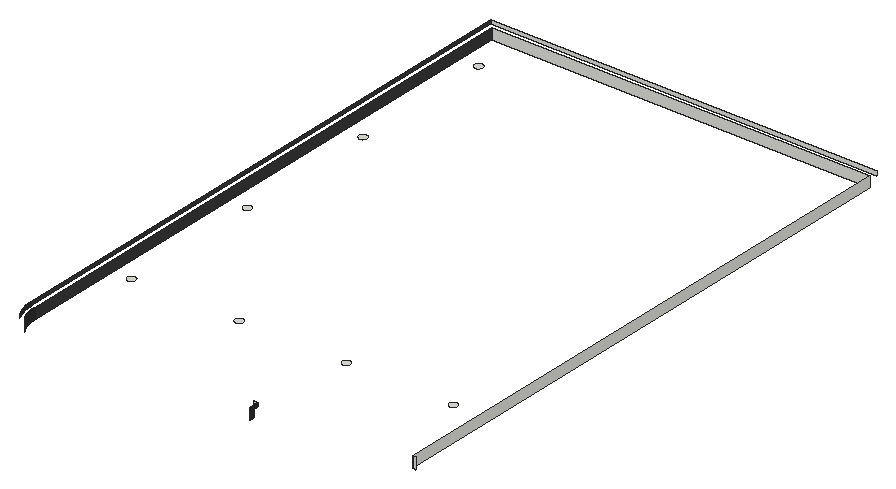
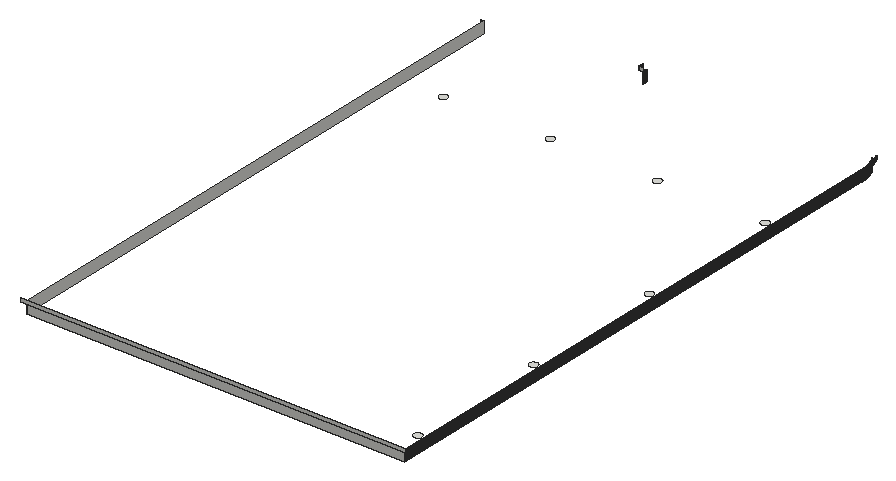
# SketchUp Ruby script. Lengths in inches.
U = 1.inch
M = Sketchup.active_model
def pt(a) = Geom::Point3d.new(a.map { |v| v * U })
def face(e, loops, mat)
  f = e.add_face(loops[0].map { |a| pt(a) })
  loops[1..].each { |l| e.add_face(l.map { |a| pt(a) }).erase! }
  f.material = f.back_material = mat if mat
  f
end
# faces: each face lists its corners as indices into pts; further lists are holes
def faces(e, pts, list, mat = nil) = list.each { |f| face(e, (f[0].is_a?(Array) ? f : [f]).map { |l| l.map { |i| pts[i] } }, mat) }
# xy, xz, yz: faces in a plane at the given z, y or x. An outline is a flat list of corners, or four numbers for a rectangle; further outlines are holes
def ring(l) = l.size == 4 ? [[l[0], l[1]], [l[2], l[1]], [l[2], l[3]], [l[0], l[3]]] : l.each_slice(2).to_a
def flat(e, list, mat, &to3) = list.each { |f| face(e, (f[0].is_a?(Array) ? f : [f]).map { |l| ring(l).map { |u, v| to3.(u, v) } }, mat) }
def xy(e, z, list, mat = nil) = flat(e, list, mat) { |x, y| [x, y, z] }
def xz(e, y, list, mat = nil) = flat(e, list, mat) { |x, z| [x, y, z] }
def yz(e, x, list, mat = nil) = flat(e, list, mat) { |y, z| [x, y, z] }
def lines(e, pts, list) = list.each { |a, b| e.add_line(pt(pts[a]), pt(pts[b])) }
# prism: a flat outline (further loops are holes) pulled along v
def prism(e, loops, v, mat = nil)
  f = face(e, loops, mat); d = Geom::Vector3d.new(v.map { |x| x * U })
  f.pushpull(f.normal.samedirection?(d) ? d.length : -d.length)
end
def box(e, o, s, mat = nil) = prism(e, [[o, [o[0] + s[0], o[1], o[2]], [o[0] + s[0], o[1] + s[1], o[2]], [o[0], o[1] + s[1], o[2]]]], [0, 0, s[2]], mat)
def at(x, y, z, deg = 0) = Geom::Transformation.translation(pt([x, y, z])) * Geom::Transformation.rotation(ORIGIN, Z_AXIS, deg.degrees)
def axes(o, x, y, z) = Geom::Transformation.new([*x, 0, *y, 0, *z, 0, *pt(o).to_a, 1])
def part(name) = M.definitions.add(name)
# library, detail: a bought-in or finely detailed component or shape, given as its bounding box
def library(name, o, s) = part(name).tap { |d| box(d.entities, o, s) }
def detail(e, o, s) = box(e.add_group.entities, o, s)
def put(e, d, t, mat = nil) = e.add_instance(d, t).tap { |i| i.material = mat if mat }
def group(e, t, mat = nil) = e.add_group.tap { |g| g.transformation = t; g.material = mat if mat }.entities
root = M.entities
M.materials.add("1496 AP 8293 CARBON COPY").color = [58, 58, 58]
xy(root,261,[[28.84,174.5,28.76,174.51,28.6875,174.52,28.61,174.53,28.45,174.55,28.375,174.57,28.3,174.58,28.22,174.6,28.15,174.625,28.07,174.65,28,174.67,27.92,174.7,27.71,174.79,27.64,174.83,27.57,174.86,27.43,174.94,27.37,174.98,27.3,175.03,27.24,175.07,27.17,175.12,26.93,175.32,26.88,175.38,26.82,175.43,26.62,175.67,26.57,175.74,26.53,175.8,26.48,175.87,26.44,175.93,26.36,176.07,26.33,176.14,26.29,176.21,26.2,176.42,26.17,176.5,26.15,176.57,26.125,176.65,26.1,176.72,26.08,176.8,26.07,176.875,26.05,176.95,26.03,177.11,26.02,177.1875,26.01,177.26,26,177.34,26,177.66,26.01,177.74,26.02,177.8125,26.03,177.89,26.05,178.05,26.07,178.125,26.08,178.2,26.1,178.28,26.125,178.35,26.15,178.43,26.17,178.5,26.2,178.58,26.29,178.79,26.33,178.86,26.36,178.93,26.44,179.07,26.48,179.13,26.53,179.2,26.57,179.26,26.62,179.33,26.82,179.57,26.88,179.62,26.93,179.68,27.17,179.88,27.24,179.93,27.3,179.97,27.37,180.02,27.43,180.06,27.57,180.14,27.64,180.17,27.71,180.21,27.92,180.3,28,180.33,28.07,180.35,28.15,180.375,28.22,180.4,28.3,180.42,28.375,180.43,28.45,180.45,28.61,180.47,28.6875,180.48,28.76,180.49,28.84,180.5,29.16,180.5,29.24,180.49,29.3125,180.48,29.39,180.47,29.55,180.45,29.625,180.43,29.7,180.42,29.78,180.4,29.85,180.375,29.93,180.35,30,180.33,30.08,180.3,30.29,180.21,30.36,180.17,30.43,180.14,30.57,180.06,30.63,180.02,30.7,179.97,30.76,179.93,30.83,179.88,31.07,179.68,31.12,179.62,31.18,179.57,31.38,179.33,31.43,179.26,31.47,179.2,31.52,179.13,31.56,179.07,31.64,178.93,31.67,178.86,31.71,178.79,31.8,178.58,31.83,178.5,31.85,178.43,31.875,178.35,31.9,178.28,31.92,178.2,31.93,178.125,31.95,178.05,31.97,177.89,31.98,177.8125,31.99,177.74,32,177.66,32,177.34,31.99,177.26,31.98,177.1875,31.97,177.11,31.95,176.95,31.93,176.875,31.92,176.8,31.9,176.72,31.875,176.65,31.85,176.57,31.83,176.5,31.8,176.42,31.71,176.21,31.67,176.14,31.64,176.07,31.56,175.93,31.52,175.87,31.47,175.8,31.43,175.74,31.38,175.67,31.18,175.43,31.12,175.38,31.07,175.32,30.83,175.12,30.76,175.07,30.7,175.03,30.63,174.98,30.57,174.94,30.43,174.86,30.36,174.83,30.29,174.79,30.08,174.7,30,174.67,29.93,174.65,29.85,174.625,29.78,174.6,29.7,174.58,29.625,174.57,29.55,174.55,29.39,174.53,29.3125,174.52,29.24,174.51,29.16,174.5],[116.51,174.5,116.35,174.52,116.28,174.53,116.12,174.55,116.04,174.57,115.97,174.58,115.89,174.6,115.81,174.625,115.74,174.65,115.67,174.67,115.59,174.7,115.45,174.76,115.375,174.79,115.3,174.83,115.24,174.86,115.03,174.98,114.97,175.03,114.9,175.07,114.6,175.32,114.55,175.38,114.49,175.43,114.4375,175.49,114.39,175.55,114.29,175.67,114.24,175.74,114.19,175.8,114.15,175.87,114.11,175.93,113.99,176.14,113.87,176.42,113.84,176.5,113.8125,176.57,113.79,176.65,113.77,176.72,113.75,176.8,113.73,176.875,113.72,176.95,113.7,177.03,113.69,177.11,113.68,177.1875,113.68,177.26,113.67,177.34,113.67,177.66,113.68,177.74,113.68,177.8125,113.69,177.89,113.7,177.97,113.72,178.05,113.73,178.125,113.75,178.2,113.77,178.28,113.79,178.35,113.8125,178.43,113.84,178.5,113.87,178.58,113.99,178.86,114.11,179.07,114.15,179.13,114.19,179.2,114.24,179.26,114.29,179.33,114.39,179.45,114.4375,179.51,114.49,179.57,114.55,179.62,114.6,179.68,114.9,179.93,114.97,179.97,115.03,180.02,115.24,180.14,115.3,180.17,115.375,180.21,115.45,180.24,115.59,180.3,115.67,180.33,115.74,180.35,115.81,180.375,115.89,180.4,115.97,180.42,116.04,180.43,116.12,180.45,116.28,180.47,116.35,180.48,116.51,180.5,116.82,180.5,117.14,180.46,117.21,180.45,117.29,180.43,117.37,180.42,117.44,180.4,117.52,180.375,117.59,180.35,117.67,180.33,117.81,180.27,117.89,180.24,117.96,180.21,118.03,180.17,118.1,180.14,118.17,180.1,118.23,180.06,118.3,180.02,118.37,179.97,118.43,179.93,118.55,179.83,118.62,179.78,118.67,179.73,118.73,179.68,118.9,179.51,119.05,179.33,119.09,179.26,119.14,179.2,119.18,179.13,119.22,179.07,119.34,178.86,119.41,178.72,119.4375,178.65,119.47,178.58,119.49,178.5,119.52,178.43,119.54,178.35,119.5625,178.28,119.58,178.2,119.62,178.05,119.64,177.89,119.65,177.8125,119.66,177.74,119.66,177.66,119.67,177.58,119.67,177.42,119.66,177.34,119.66,177.26,119.65,177.1875,119.64,177.11,119.62,176.95,119.58,176.8,119.5625,176.72,119.54,176.65,119.52,176.57,119.49,176.5,119.47,176.42,119.4375,176.35,119.41,176.28,119.34,176.14,119.22,175.93,119.18,175.87,119.14,175.8,119.09,175.74,119.05,175.67,118.9,175.49,118.73,175.32,118.67,175.27,118.62,175.22,118.55,175.17,118.43,175.07,118.37,175.03,118.3,174.98,118.23,174.94,118.17,174.9,118.1,174.86,118.03,174.83,117.96,174.79,117.89,174.76,117.81,174.73,117.67,174.67,117.59,174.65,117.52,174.625,117.44,174.6,117.37,174.58,117.29,174.57,117.21,174.55,117.14,174.54,116.82,174.5],[204.18,174.5,203.86,174.54,203.79,174.55,203.71,174.57,203.63,174.58,203.56,174.6,203.48,174.625,203.41,174.65,203.33,174.67,203.19,174.73,203.11,174.76,203.04,174.79,202.97,174.83,202.9,174.86,202.83,174.9,202.77,174.94,202.7,174.98,202.63,175.03,202.57,175.07,202.45,175.17,202.38,175.22,202.33,175.27,202.27,175.32,202.1,175.49,201.95,175.67,201.91,175.74,201.86,175.8,201.82,175.87,201.78,175.93,201.66,176.14,201.59,176.28,201.5625,176.35,201.53,176.42,201.51,176.5,201.48,176.57,201.46,176.65,201.4375,176.72,201.42,176.8,201.38,176.95,201.36,177.11,201.35,177.1875,201.34,177.26,201.34,177.34,201.33,177.42,201.33,177.58,201.34,177.66,201.34,177.74,201.35,177.8125,201.36,177.89,201.38,178.05,201.42,178.2,201.4375,178.28,201.46,178.35,201.48,178.43,201.51,178.5,201.53,178.58,201.5625,178.65,201.59,178.72,201.66,178.86,201.78,179.07,201.82,179.13,201.86,179.2,201.91,179.26,201.95,179.33,202.1,179.51,202.27,179.68,202.33,179.73,202.38,179.78,202.45,179.83,202.57,179.93,202.63,179.97,202.7,180.02,202.77,180.06,202.83,180.1,202.9,180.14,202.97,180.17,203.04,180.21,203.11,180.24,203.19,180.27,203.33,180.33,203.41,180.35,203.48,180.375,203.56,180.4,203.63,180.42,203.71,180.43,203.79,180.45,203.86,180.46,204.18,180.5,204.49,180.5,204.65,180.48,204.72,180.47,204.88,180.45,204.96,180.43,205.03,180.42,205.11,180.4,205.19,180.375,205.26,180.35,205.33,180.33,205.41,180.3,205.55,180.24,205.625,180.21,205.7,180.17,205.76,180.14,205.97,180.02,206.03,179.97,206.1,179.93,206.4,179.68,206.45,179.62,206.51,179.57,206.5625,179.51,206.61,179.45,206.71,179.33,206.76,179.26,206.81,179.2,206.85,179.13,206.89,179.07,207.01,178.86,207.13,178.58,207.16,178.5,207.1875,178.43,207.21,178.35,207.23,178.28,207.25,178.2,207.27,178.125,207.28,178.05,207.3,177.97,207.31,177.89,207.32,177.8125,207.32,177.74,207.33,177.66,207.33,177.34,207.32,177.26,207.32,177.1875,207.31,177.11,207.3,177.03,207.28,176.95,207.27,176.875,207.25,176.8,207.23,176.72,207.21,176.65,207.1875,176.57,207.16,176.5,207.13,176.42,207.01,176.14,206.89,175.93,206.85,175.87,206.81,175.8,206.76,175.74,206.71,175.67,206.61,175.55,206.5625,175.49,206.51,175.43,206.45,175.38,206.4,175.32,206.1,175.07,206.03,175.03,205.97,174.98,205.76,174.86,205.7,174.83,205.625,174.79,205.55,174.76,205.41,174.7,205.33,174.67,205.26,174.65,205.19,174.625,205.11,174.6,205.03,174.58,204.96,174.57,204.88,174.55,204.72,174.53,204.65,174.52,204.49,174.5],[291.84,174.5,291.76,174.51,291.6875,174.52,291.61,174.53,291.45,174.55,291.375,174.57,291.3,174.58,291.22,174.6,291.15,174.625,291.07,174.65,291,174.67,290.92,174.7,290.71,174.79,290.64,174.83,290.57,174.86,290.43,174.94,290.37,174.98,290.3,175.03,290.24,175.07,290.17,175.12,289.93,175.32,289.88,175.38,289.82,175.43,289.62,175.67,289.57,175.74,289.53,175.8,289.48,175.87,289.44,175.93,289.36,176.07,289.33,176.14,289.29,176.21,289.2,176.42,289.17,176.5,289.15,176.57,289.125,176.65,289.1,176.72,289.08,176.8,289.07,176.875,289.05,176.95,289.03,177.11,289.02,177.1875,289.01,177.26,289,177.34,289,177.66,289.01,177.74,289.02,177.8125,289.03,177.89,289.05,178.05,289.07,178.125,289.08,178.2,289.1,178.28,289.125,178.35,289.15,178.43,289.17,178.5,289.2,178.58,289.29,178.79,289.33,178.86,289.36,178.93,289.44,179.07,289.48,179.13,289.53,179.2,289.57,179.26,289.62,179.33,289.82,179.57,289.88,179.62,289.93,179.68,290.17,179.88,290.24,179.93,290.3,179.97,290.37,180.02,290.43,180.06,290.57,180.14,290.64,180.17,290.71,180.21,290.92,180.3,291,180.33,291.07,180.35,291.15,180.375,291.22,180.4,291.3,180.42,291.375,180.43,291.45,180.45,291.61,180.47,291.6875,180.48,291.76,180.49,291.84,180.5,292.16,180.5,292.24,180.49,292.3125,180.48,292.39,180.47,292.55,180.45,292.625,180.43,292.7,180.42,292.78,180.4,292.85,180.375,292.93,180.35,293,180.33,293.08,180.3,293.29,180.21,293.36,180.17,293.43,180.14,293.57,180.06,293.63,180.02,293.7,179.97,293.76,179.93,293.83,179.88,294.07,179.68,294.12,179.62,294.18,179.57,294.38,179.33,294.43,179.26,294.47,179.2,294.52,179.13,294.56,179.07,294.64,178.93,294.67,178.86,294.71,178.79,294.8,178.58,294.83,178.5,294.85,178.43,294.875,178.35,294.9,178.28,294.92,178.2,294.93,178.125,294.95,178.05,294.97,177.89,294.98,177.8125,294.99,177.74,295,177.66,295,177.34,294.99,177.26,294.98,177.1875,294.97,177.11,294.95,176.95,294.93,176.875,294.92,176.8,294.9,176.72,294.875,176.65,294.85,176.57,294.83,176.5,294.8,176.42,294.71,176.21,294.67,176.14,294.64,176.07,294.56,175.93,294.52,175.87,294.47,175.8,294.43,175.74,294.38,175.67,294.18,175.43,294.12,175.38,294.07,175.32,293.83,175.12,293.76,175.07,293.7,175.03,293.63,174.98,293.57,174.94,293.43,174.86,293.36,174.83,293.29,174.79,293.08,174.7,293,174.67,292.93,174.65,292.85,174.625,292.78,174.6,292.7,174.58,292.625,174.57,292.55,174.55,292.39,174.53,292.3125,174.52,292.24,174.51,292.16,174.5],[28.84,292.67,28.76,292.68,28.6875,292.68,28.61,292.69,28.53,292.7,28.45,292.72,28.375,292.73,28.3,292.75,28.22,292.77,28.15,292.79,28.07,292.8125,28,292.84,27.92,292.87,27.64,292.99,27.43,293.11,27.37,293.15,27.3,293.19,27.24,293.24,27.17,293.29,27.05,293.39,26.99,293.4375,26.93,293.49,26.88,293.55,26.82,293.6,26.57,293.9,26.53,293.97,26.48,294.03,26.36,294.24,26.33,294.3,26.29,294.375,26.26,294.45,26.2,294.59,26.17,294.67,26.15,294.74,26.125,294.81,26.1,294.89,26.08,294.97,26.07,295.04,26.05,295.12,26.03,295.28,26.02,295.35,26,295.51,26,295.82,26.04,296.14,26.05,296.21,26.07,296.29,26.08,296.37,26.1,296.44,26.125,296.52,26.15,296.59,26.17,296.67,26.23,296.81,26.26,296.89,26.29,296.96,26.33,297.03,26.36,297.1,26.4,297.17,26.44,297.23,26.48,297.3,26.53,297.37,26.57,297.43,26.67,297.55,26.72,297.62,26.77,297.67,26.82,297.73,26.99,297.9,27.17,298.05,27.24,298.09,27.3,298.14,27.37,298.18,27.43,298.22,27.64,298.34,27.78,298.41,27.85,298.4375,27.92,298.47,28,298.49,28.07,298.52,28.15,298.54,28.22,298.5625,28.3,298.58,28.45,298.62,28.61,298.64,28.6875,298.65,28.76,298.66,28.84,298.66,28.92,298.67,29.08,298.67,29.16,298.66,29.24,298.66,29.3125,298.65,29.39,298.64,29.55,298.62,29.7,298.58,29.78,298.5625,29.85,298.54,29.93,298.52,30,298.49,30.08,298.47,30.15,298.4375,30.22,298.41,30.36,298.34,30.57,298.22,30.63,298.18,30.7,298.14,30.76,298.09,30.83,298.05,31.01,297.9,31.18,297.73,31.23,297.67,31.28,297.62,31.33,297.55,31.43,297.43,31.47,297.37,31.52,297.3,31.56,297.23,31.6,297.17,31.64,297.1,31.67,297.03,31.71,296.96,31.74,296.89,31.77,296.81,31.83,296.67,31.85,296.59,31.875,296.52,31.9,296.44,31.92,296.37,31.93,296.29,31.95,296.21,31.96,296.14,32,295.82,32,295.51,31.98,295.35,31.97,295.28,31.95,295.12,31.93,295.04,31.92,294.97,31.9,294.89,31.875,294.81,31.85,294.74,31.83,294.67,31.8,294.59,31.74,294.45,31.71,294.375,31.67,294.3,31.64,294.24,31.52,294.03,31.47,293.97,31.43,293.9,31.18,293.6,31.12,293.55,31.07,293.49,31.01,293.4375,30.95,293.39,30.83,293.29,30.76,293.24,30.7,293.19,30.63,293.15,30.57,293.11,30.36,292.99,30.08,292.87,30,292.84,29.93,292.8125,29.85,292.79,29.78,292.77,29.7,292.75,29.625,292.73,29.55,292.72,29.47,292.7,29.39,292.69,29.3125,292.68,29.24,292.68,29.16,292.67],
  [28.92,410.83,28.84,410.84,28.76,410.84,28.6875,410.85,28.61,410.86,28.45,410.88,28.3,410.92,28.22,410.9375,28.15,410.96,28.07,410.98,28,411.01,27.92,411.03,27.85,411.0625,27.78,411.09,27.64,411.16,27.43,411.28,27.37,411.32,27.3,411.36,27.24,411.41,27.17,411.45,26.99,411.6,26.82,411.77,26.77,411.83,26.72,411.88,26.67,411.95,26.57,412.07,26.53,412.13,26.48,412.2,26.44,412.27,26.4,412.33,26.36,412.4,26.33,412.47,26.29,412.54,26.26,412.61,26.23,412.69,26.17,412.83,26.15,412.91,26.125,412.98,26.1,413.06,26.08,413.13,26.07,413.21,26.05,413.29,26.04,413.36,26,413.68,26,413.99,26.02,414.15,26.03,414.22,26.05,414.38,26.07,414.46,26.08,414.53,26.1,414.61,26.125,414.69,26.15,414.76,26.17,414.83,26.2,414.91,26.26,415.05,26.29,415.125,26.33,415.2,26.36,415.26,26.48,415.47,26.53,415.53,26.57,415.6,26.82,415.9,26.88,415.95,26.93,416.01,26.99,416.0625,27.05,416.11,27.17,416.21,27.24,416.26,27.3,416.31,27.37,416.35,27.43,416.39,27.64,416.51,27.92,416.63,28,416.66,28.07,416.6875,28.15,416.71,28.22,416.73,28.3,416.75,28.375,416.77,28.45,416.78,28.53,416.8,28.61,416.81,28.6875,416.82,28.76,416.82,28.84,416.83,29.16,416.83,29.24,416.82,29.3125,416.82,29.39,416.81,29.47,416.8,29.55,416.78,29.625,416.77,29.7,416.75,29.78,416.73,29.85,416.71,29.93,416.6875,30,416.66,30.08,416.63,30.36,416.51,30.57,416.39,30.63,416.35,30.7,416.31,30.76,416.26,30.83,416.21,30.95,416.11,31.01,416.0625,31.07,416.01,31.12,415.95,31.18,415.9,31.43,415.6,31.47,415.53,31.52,415.47,31.64,415.26,31.67,415.2,31.71,415.125,31.74,415.05,31.8,414.91,31.83,414.83,31.85,414.76,31.875,414.69,31.9,414.61,31.92,414.53,31.93,414.46,31.95,414.38,31.97,414.22,31.98,414.15,32,413.99,32,413.68,31.96,413.36,31.95,413.29,31.93,413.21,31.92,413.13,31.9,413.06,31.875,412.98,31.85,412.91,31.83,412.83,31.77,412.69,31.74,412.61,31.71,412.54,31.67,412.47,31.64,412.4,31.6,412.33,31.56,412.27,31.52,412.2,31.47,412.13,31.43,412.07,31.33,411.95,31.28,411.88,31.23,411.83,31.18,411.77,31.01,411.6,30.83,411.45,30.76,411.41,30.7,411.36,30.63,411.32,30.57,411.28,30.36,411.16,30.22,411.09,30.15,411.0625,30.08,411.03,30,411.01,29.93,410.98,29.85,410.96,29.78,410.9375,29.7,410.92,29.55,410.88,29.39,410.86,29.3125,410.85,29.24,410.84,29.16,410.84,29.08,410.83],[28.84,529,28.76,529.01,28.6875,529.02,28.61,529.03,28.45,529.05,28.375,529.07,28.3,529.08,28.22,529.1,28.15,529.125,28.07,529.15,28,529.17,27.92,529.2,27.71,529.29,27.64,529.33,27.57,529.36,27.43,529.44,27.37,529.48,27.3,529.53,27.24,529.57,27.17,529.62,26.93,529.82,26.88,529.88,26.82,529.93,26.62,530.17,26.57,530.24,26.53,530.3,26.48,530.37,26.44,530.43,26.36,530.57,26.33,530.64,26.29,530.71,26.2,530.92,26.17,531,26.15,531.07,26.125,531.15,26.1,531.22,26.08,531.3,26.07,531.375,26.05,531.45,26.03,531.61,26.02,531.6875,26.01,531.76,26,531.84,26,532.16,26.01,532.24,26.02,532.3125,26.03,532.39,26.05,532.55,26.07,532.625,26.08,532.7,26.1,532.78,26.125,532.85,26.15,532.93,26.17,533,26.2,533.08,26.29,533.29,26.33,533.36,26.36,533.43,26.44,533.57,26.48,533.63,26.53,533.7,26.57,533.76,26.62,533.83,26.82,534.07,26.88,534.12,26.93,534.18,27.17,534.38,27.24,534.43,27.3,534.47,27.37,534.52,27.43,534.56,27.57,534.64,27.64,534.67,27.71,534.71,27.92,534.8,28,534.83,28.07,534.85,28.15,534.875,28.22,534.9,28.3,534.92,28.375,534.93,28.45,534.95,28.61,534.97,28.6875,534.98,28.76,534.99,28.84,535,29.16,535,29.24,534.99,29.3125,534.98,29.39,534.97,29.55,534.95,29.625,534.93,29.7,534.92,29.78,534.9,29.85,534.875,29.93,534.85,30,534.83,30.08,534.8,30.29,534.71,30.36,534.67,30.43,534.64,30.57,534.56,30.63,534.52,30.7,534.47,30.76,534.43,30.83,534.38,31.07,534.18,31.12,534.12,31.18,534.07,31.38,533.83,31.43,533.76,31.47,533.7,31.52,533.63,31.56,533.57,31.64,533.43,31.67,533.36,31.71,533.29,31.8,533.08,31.83,533,31.85,532.93,31.875,532.85,31.9,532.78,31.92,532.7,31.93,532.625,31.95,532.55,31.97,532.39,31.98,532.3125,31.99,532.24,32,532.16,32,531.84,31.99,531.76,31.98,531.6875,31.97,531.61,31.95,531.45,31.93,531.375,31.92,531.3,31.9,531.22,31.875,531.15,31.85,531.07,31.83,531,31.8,530.92,31.71,530.71,31.67,530.64,31.64,530.57,31.56,530.43,31.52,530.37,31.47,530.3,31.43,530.24,31.38,530.17,31.18,529.93,31.12,529.88,31.07,529.82,30.83,529.62,30.76,529.57,30.7,529.53,30.63,529.48,30.57,529.44,30.43,529.36,30.36,529.33,30.29,529.29,30.08,529.2,30,529.17,29.93,529.15,29.85,529.125,29.78,529.1,29.7,529.08,29.625,529.07,29.55,529.05,29.39,529.03,29.3125,529.02,29.24,529.01,29.16,529]])
xz(root,85,[[203,270,206,273]])
xz(root,97,[[323,261,326,270]])
xz(root,564,[[14,261,323,270]])
xz(root,567,[[11,270,326,273]])
yz(root,11,[[96.57,270,97,273],[97,270,567,273]],"1496 AP 8293 CARBON COPY")
yz(root,14,[[96.61,261,97,270],[97,261,564,270]],"1496 AP 8293 CARBON COPY")
yz(root,202.99,[[84.29,261,84.53,270]],"1496 AP 8293 CARBON COPY")
yz(root,203,[[84.76,261,85,270]],"1496 AP 8293 CARBON COPY")
yz(root,206,[[84.73,270,85,273]],"1496 AP 8293 CARBON COPY")
yz(root,323,[[97,261,564,270]])
p = [[18.63,80.99,261],[18.63,80.99,270],[18.42,81.33,270],[18.42,81.33,261],[18.22,81.66,270],[18.22,81.66,261],
  [202.65,81.49,261],[202.65,81.49,270],[202.61,81.26,270],[202.61,81.26,261],[202.7,81.72,261],[202.7,81.72,270],
  [18.02,82,270],[18.02,82,261],[202.74,81.95,261],[202.74,81.95,270],[17.83,82.34,270],[17.83,82.34,261],
  [202.78,82.18,261],[202.78,82.18,270],[202.8125,82.42,261],[202.8125,82.42,270],[17.64,82.69,270],[17.64,82.69,261],
  [202.85,82.65,261],[202.85,82.65,270],[17.45,83.03,270],[17.45,83.03,261],[202.875,82.88,261],[202.875,82.88,270],
  [202.9,83.12,261],[202.9,83.12,270],[17.27,83.38,270],[17.27,83.38,261],[202.92,83.35,261],[202.92,83.35,270],
  [17.09,83.73,270],[17.09,83.73,261],[202.94,83.59,261],[202.94,83.59,270],[202.96,83.82,261],[202.96,83.82,270],
  [16.92,84.08,270],[16.92,84.08,261],[202.98,84.06,261],[202.98,84.06,270],[16.76,84.44,270],[16.76,84.44,261],
  [202.99,84.29,261],[202.99,84.29,270],[16.59,84.8,270],[16.59,84.8,261],[203,84.76,261],[203,84.76,270],
  [202.99,84.53,270],[202.99,84.53,261],[16.4375,85.16,270],[16.4375,85.16,261],[16.28,85.52,270],[16.28,85.52,261],
  [16.14,85.88,270],[16.14,85.88,261],[15.99,86.25,270],[15.99,86.25,261],[15.85,86.62,270],[15.85,86.62,261],
  [15.72,86.99,270],[15.72,86.99,261],[15.59,87.36,270],[15.59,87.36,261],[15.47,87.73,270],[15.47,87.73,261],
  [15.35,88.1,270],[15.35,88.1,261],[15.24,88.48,270],[15.24,88.48,261],[15.125,88.86,270],[15.125,88.86,261],
  [15.02,89.24,270],[15.02,89.24,261],[14.92,89.62,270],[14.92,89.62,261],[14.83,90,270],[14.83,90,261],
  [14.74,90.38,270],[14.74,90.38,261],[14.66,90.76,270],[14.66,90.76,261],[14.58,91.15,270],[14.58,91.15,261],
  [14.5,91.53,270],[14.5,91.53,261],[14.43,91.92,270],[14.43,91.92,261],[14.37,92.31,270],[14.37,92.31,261],
  [14.31,92.7,270],[14.31,92.7,261],[14.26,93.08,270],[14.26,93.08,261],[14.21,93.47,270],[14.21,93.47,261],
  [14.16,93.86,270],[14.16,93.86,261],[14.125,94.25,270],[14.125,94.25,261],[14.09,94.65,270],[14.09,94.65,261],
  [14.0625,95.04,270],[14.0625,95.04,261],[14.04,95.43,270],[14.04,95.43,261],[14.02,95.82,270],[14.02,95.82,261],
  [14.01,96.21,270],[14.01,96.21,261],[14,96.61,270],[14,96.61,261],[205.65,81.17,270],[205.7,81.44,270],
  [205.7,81.44,273],[205.65,81.17,273],[14.8,81.63,270],[15,81.25,270],[15,81.25,273],[14.8,81.63,273],
  [205.74,81.71,270],[205.74,81.71,273],[14.6,82.02,270],[14.6,82.02,273],[205.78,81.99,270],[205.78,81.99,273],
  [14.4,82.4,270],[14.4,82.4,273],[205.82,82.26,270],[205.82,82.26,273],[205.85,82.53,270],[205.85,82.53,273],
  [14.21,82.79,270],[14.21,82.79,273],[205.88,82.8,270],[205.88,82.8,273],[14.03,83.18,270],[14.03,83.18,273],
  [205.91,83.08,270],[205.91,83.08,273],[205.94,83.35,270],[205.94,83.35,273],[13.85,83.58,270],[13.85,83.58,273],
  [205.96,83.625,270],[205.96,83.625,273],[13.68,83.97,270],[13.68,83.97,273],[205.97,83.9,270],[205.97,83.9,273],
  [205.98,84.18,270],[205.98,84.18,273],[13.51,84.37,270],[13.51,84.37,273],[205.99,84.45,270],[205.99,84.45,273],
  [13.35,84.77,270],[13.35,84.77,273],[206,84.73,270],[206,84.73,273],[13.19,85.17,270],[13.19,85.17,273],
  [13.04,85.58,270],[13.04,85.58,273],[12.89,85.98,270],[12.89,85.98,273],[12.75,86.39,270],[12.75,86.39,273],
  [12.62,86.8,270],[12.62,86.8,273],[12.48,87.21,270],[12.48,87.21,273],[12.36,87.63,270],[12.36,87.63,273],
  [12.24,88.04,270],[12.24,88.04,273],[12.125,88.46,270],[12.125,88.46,273],[12.02,88.875,270],[12.02,88.875,273],
  [11.91,89.3,270],[11.91,89.3,273],[11.8125,89.72,270],[11.8125,89.72,273],[11.72,90.14,270],[11.72,90.14,273],
  [11.63,90.5625,270],[11.63,90.5625,273],[11.55,90.99,270],[11.55,90.99,273],[11.48,91.41,270],[11.48,91.41,273],
  [11.41,91.84,270],[11.41,91.84,273],[11.34,92.26,270],[11.34,92.26,273],[11.28,92.69,270],[11.28,92.69,273],
  [11.23,93.12,270],[11.23,93.12,273],[11.18,93.55,270],[11.18,93.55,273],[11.14,93.98,270],[11.14,93.98,273],
  [11.1,94.41,270],[11.1,94.41,273],[11.07,94.84,270],[11.07,94.84,273],[11.05,95.27,270],[11.05,95.27,273],
  [11.03,95.7,270],[11.03,95.7,273],[11.01,96.14,270],[11.01,96.14,273],[11,96.57,270],[11,96.57,273],
  [323,94,270],[323,94,273]]
faces(root,p,[[0,1,2,3],[3,2,4,5],[6,7,8,9],[10,11,7,6],[5,4,12,13],[14,15,11,10],[13,12,16,17],[18,19,15,14],
  [20,21,19,18],[17,16,22,23],[24,25,21,20],[23,22,26,27],[28,29,25,24],[30,31,29,28],[27,26,32,33],[34,35,31,30],
  [33,32,36,37],[38,39,35,34],[40,41,39,38],[37,36,42,43],[44,45,41,40],[43,42,46,47],[48,49,45,44],[47,46,50,51],
  [52,53,54,55],[51,50,56,57],[57,56,58,59],[59,58,60,61],[61,60,62,63],[63,62,64,65],[65,64,66,67],[67,66,68,69],
  [69,68,70,71],[71,70,72,73],[73,72,74,75],[75,74,76,77],[77,76,78,79],[79,78,80,81],[81,80,82,83],[83,82,84,85],
  [85,84,86,87],[87,86,88,89],[89,88,90,91],[91,90,92,93],[93,92,94,95],[95,94,96,97],[97,96,98,99],[99,98,100,101],
  [101,100,102,103],[103,102,104,105],[105,104,106,107],[107,106,108,109],[109,108,110,111],[111,110,112,113],[113,112,114,115],[115,114,116,117],
  [118,119,120,121],[122,123,124,125],[119,126,127,120],[128,122,125,129],[126,130,131,127],[132,128,129,133],[130,134,135,131],[134,136,137,135],
  [138,132,133,139],[136,140,141,137],[142,138,139,143],[140,144,145,141],[144,146,147,145],[148,142,143,149],[146,150,151,147],[152,148,149,153],
  [150,154,155,151],[154,156,157,155],[158,152,153,159],[156,160,161,157],[162,158,159,163],[160,164,165,161],[166,162,163,167],[168,166,167,169],
  [170,168,169,171],[172,170,171,173],[174,172,173,175],[176,174,175,177],[178,176,177,179],[180,178,179,181],[182,180,181,183],[184,182,183,185],
  [186,184,185,187],[188,186,187,189],[190,188,189,191],[192,190,191,193],[194,192,193,195],[196,194,195,197],[198,196,197,199],[200,198,199,201],
  [202,200,201,203],[204,202,203,205],[206,204,205,207],[208,206,207,209],[210,208,209,211],[212,210,211,213],[214,212,213,215],[216,214,215,217],
  [218,216,217,219],[220,218,219,221]],"1496 AP 8293 CARBON COPY")
lines(root,p,[[222,223]])
